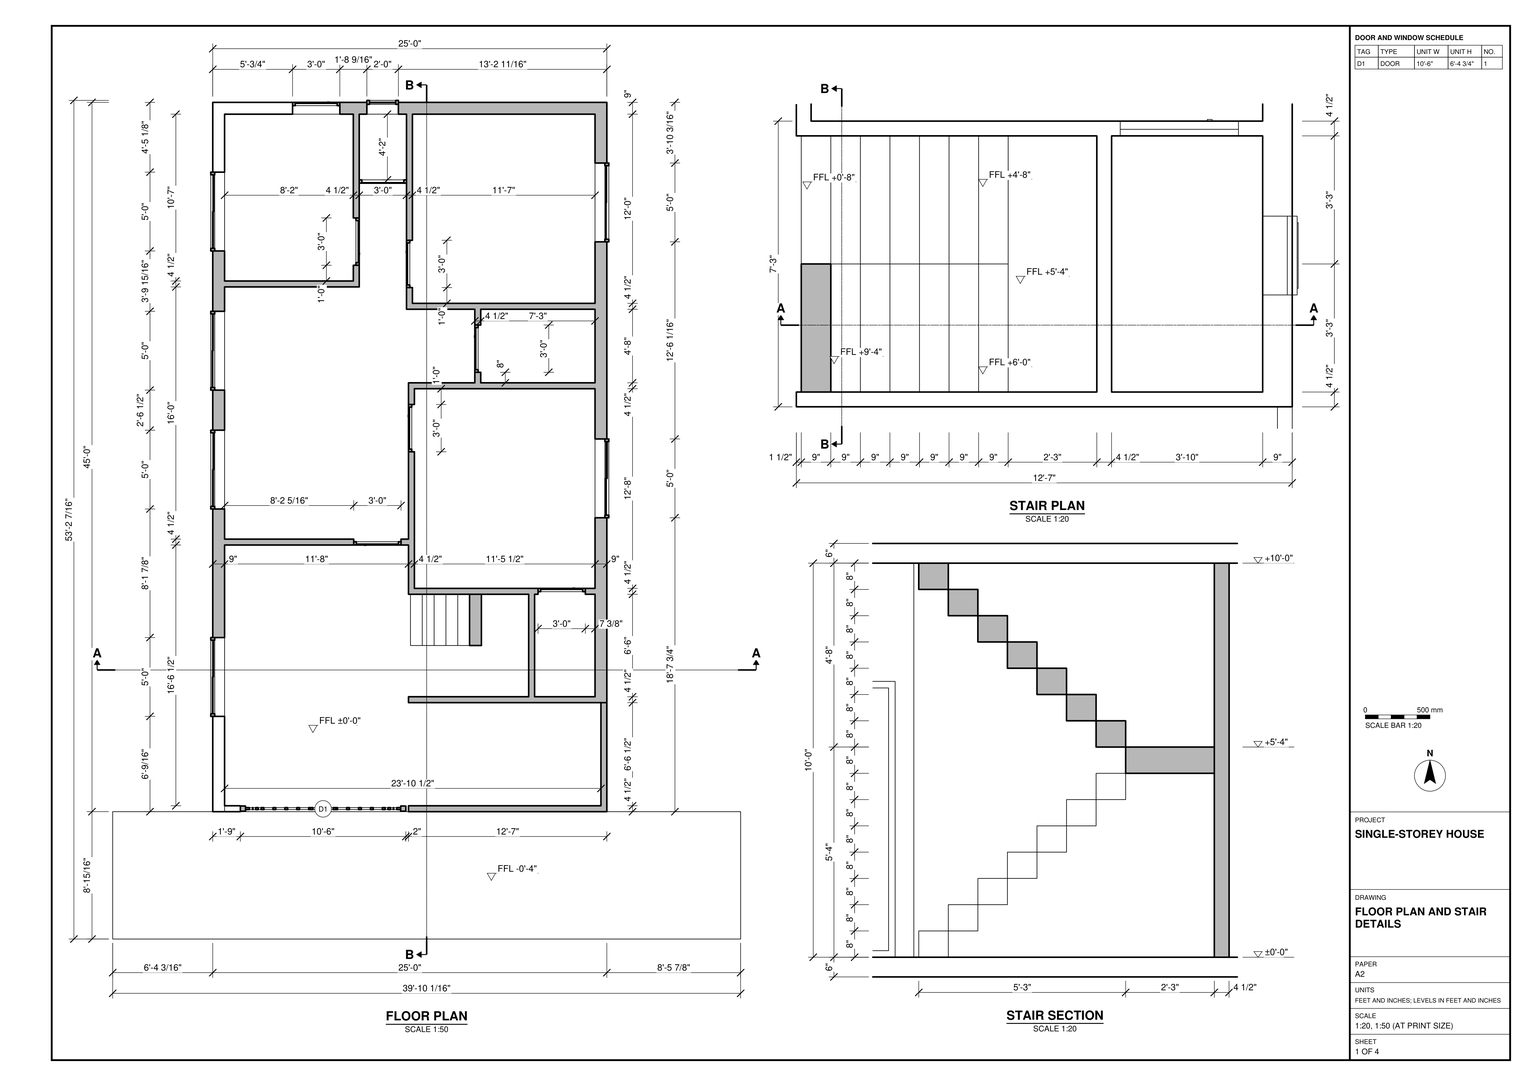
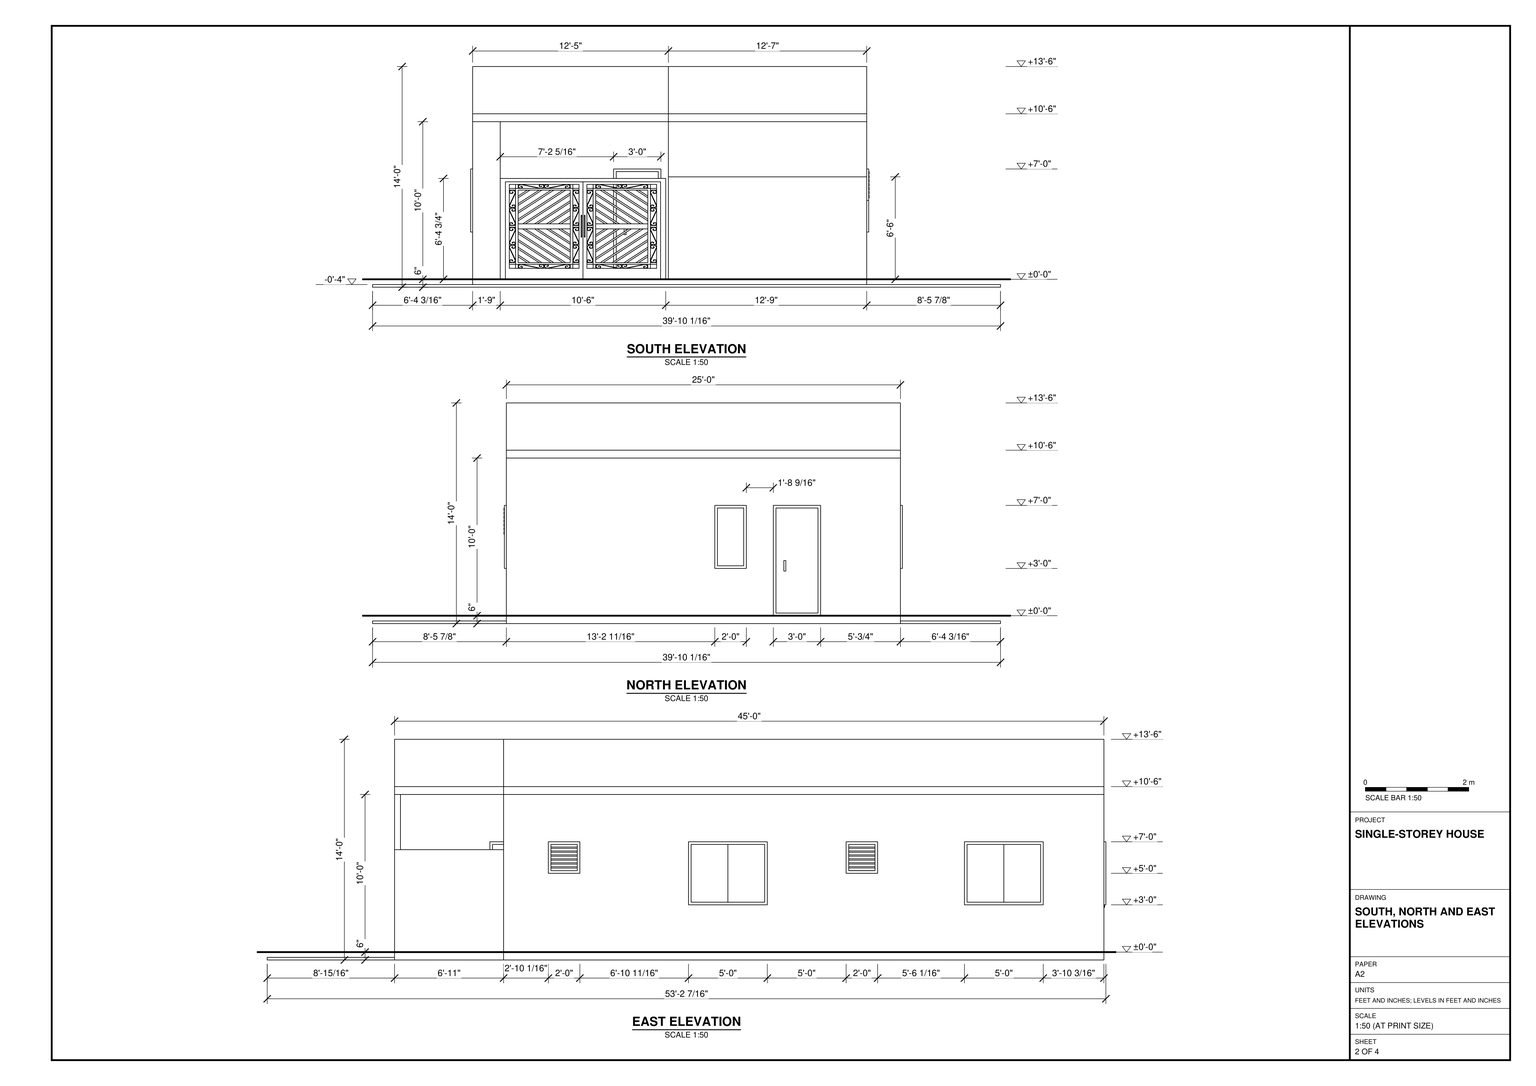
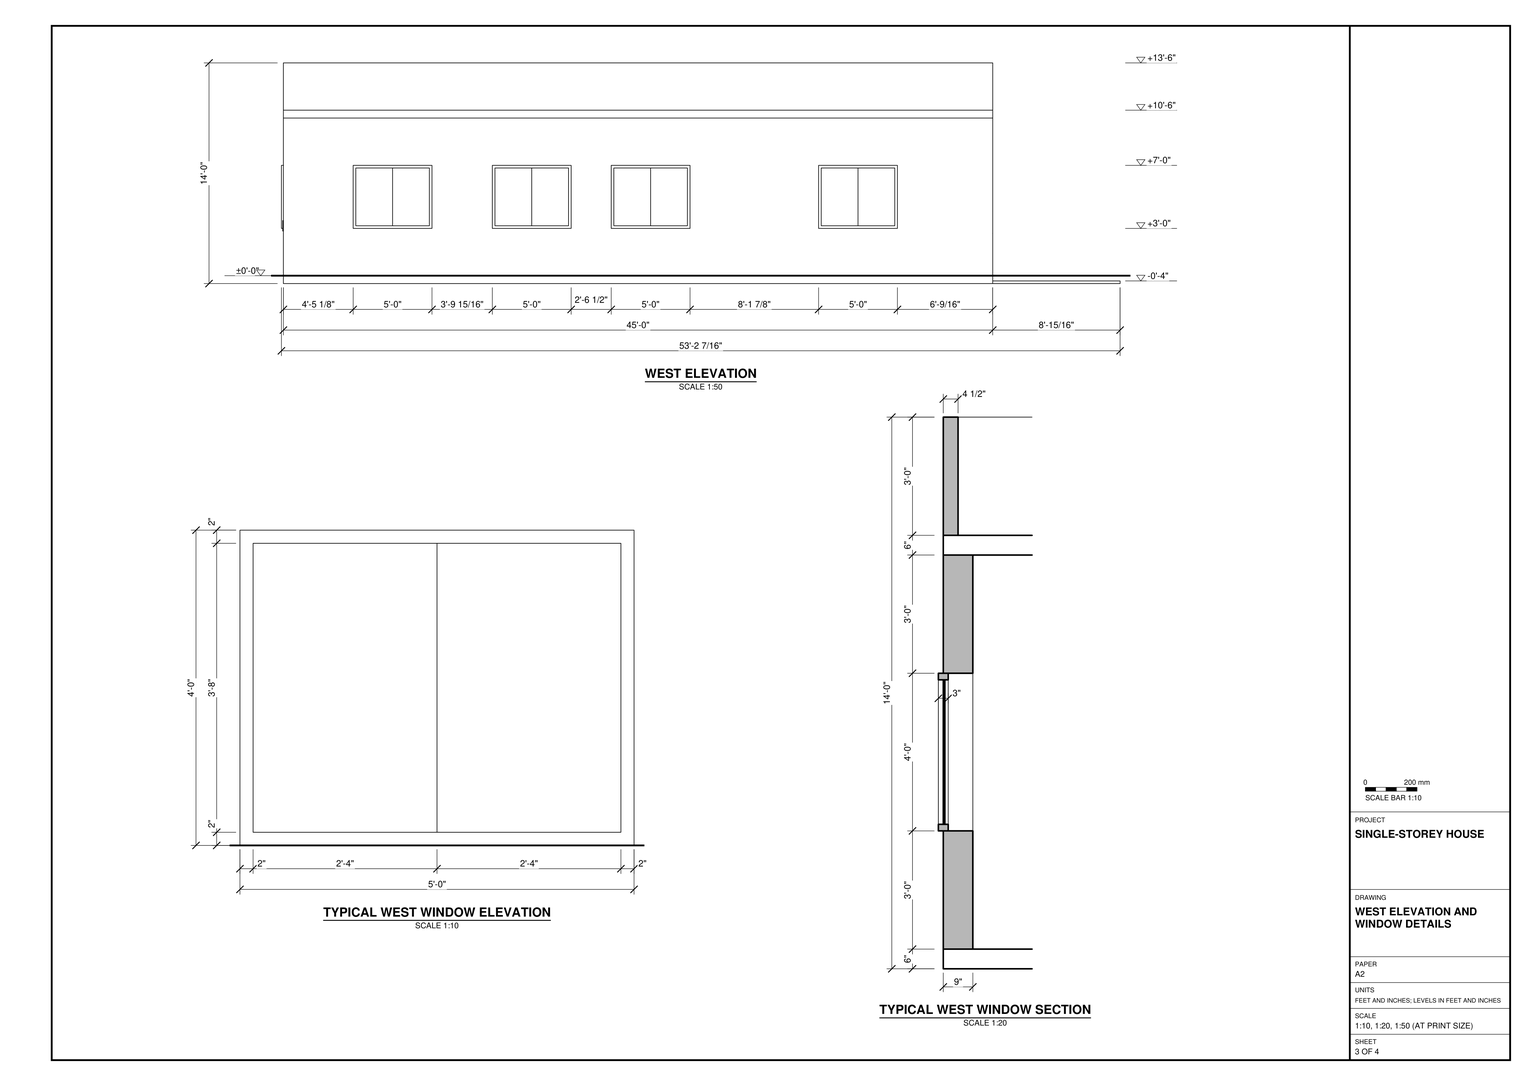
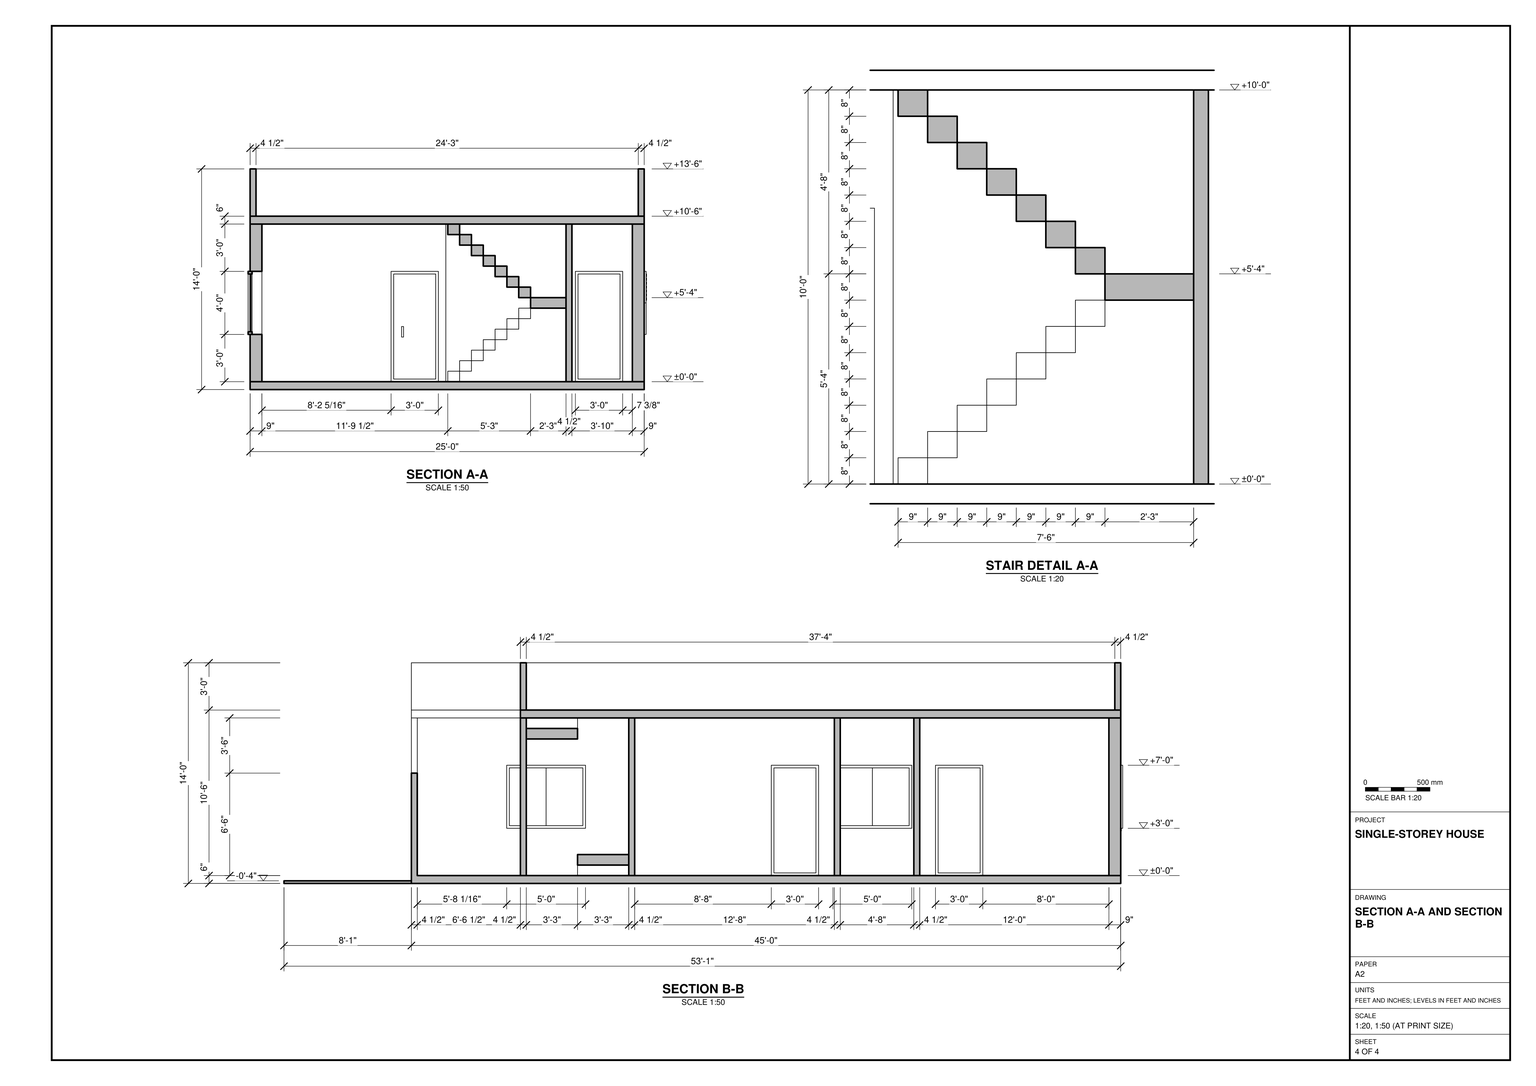
Build the single-storey house in SketchUp from task_files/diagram_01.pdf. Work in feet and inches. Set the ground floor at ±0'-0". The complete model, including the apron outside the south entrance, measures 39'-10 1/16" east to west, 53'-2 7/16" north to south and 14'-0" high. The house itself has a 25'-0" by 45'-0" footprint. Set the apron surface at -0'-4" and extend it past both sides of the house as shown in plan.

Model the floor slab, exterior walls and interior partitions, following the thicknesses and doorway positions on the plan. Preserve the open entrance area, the stair near its east side and the passage connecting the rooms farther north. Build the two stair flights and their intermediate landing from the stair plan and section. Model the flat roof slab and raised perimeter parapet. Fit the south entrance with the paired gate leaves shown in elevation. Use the window detail for the divided west windows, and distinguish the smaller louvred openings from the larger glazed windows on the east wall.

Keep shell elements such as walls, slabs and roof, and each furniture or joinery piece shown, in separate groups or components; use components for repeated parts. Any decor or loose items shown may be suitable library components. Save one SketchUp model as output_files/gated_single_storey_house_with_return_stair.skp.

# SketchUp Ruby script. Lengths in inches.
U = 1.inch
M = Sketchup.active_model
def pt(a) = Geom::Point3d.new(a.map { |v| v * U })
def face(e, loops, mat)
  f = e.add_face(loops[0].map { |a| pt(a) })
  loops[1..].each { |l| e.add_face(l.map { |a| pt(a) }).erase! }
  f.material = f.back_material = mat if mat
  f
end
# faces: each face lists its corners as indices into pts; further lists are holes
def faces(e, pts, list, mat = nil) = list.each { |f| face(e, (f[0].is_a?(Array) ? f : [f]).map { |l| l.map { |i| pts[i] } }, mat) }
# xy, xz, yz: faces in a plane at the given z, y or x. An outline is a flat list of corners, or four numbers for a rectangle; further outlines are holes
def ring(l) = l.size == 4 ? [[l[0], l[1]], [l[2], l[1]], [l[2], l[3]], [l[0], l[3]]] : l.each_slice(2).to_a
def flat(e, list, mat, &to3) = list.each { |f| face(e, (f[0].is_a?(Array) ? f : [f]).map { |l| ring(l).map { |u, v| to3.(u, v) } }, mat) }
def xy(e, z, list, mat = nil) = flat(e, list, mat) { |x, y| [x, y, z] }
def xz(e, y, list, mat = nil) = flat(e, list, mat) { |x, z| [x, y, z] }
def yz(e, x, list, mat = nil) = flat(e, list, mat) { |y, z| [x, y, z] }
def lines(e, pts, list) = list.each { |a, b| e.add_line(pt(pts[a]), pt(pts[b])) }
# prism: a flat outline (further loops are holes) pulled along v
def prism(e, loops, v, mat = nil)
  f = face(e, loops, mat); d = Geom::Vector3d.new(v.map { |x| x * U })
  f.pushpull(f.normal.samedirection?(d) ? d.length : -d.length)
end
def box(e, o, s, mat = nil) = prism(e, [[o, [o[0] + s[0], o[1], o[2]], [o[0] + s[0], o[1] + s[1], o[2]], [o[0], o[1] + s[1], o[2]]]], [0, 0, s[2]], mat)
def at(x, y, z, deg = 0) = Geom::Transformation.translation(pt([x, y, z])) * Geom::Transformation.rotation(ORIGIN, Z_AXIS, deg.degrees)
def axes(o, x, y, z) = Geom::Transformation.new([*x, 0, *y, 0, *z, 0, *pt(o).to_a, 1])
def part(name) = M.definitions.add(name)
# library, detail: a bought-in or finely detailed component or shape, given as its bounding box
def library(name, o, s) = part(name).tap { |d| box(d.entities, o, s) }
def detail(e, o, s) = box(e.add_group.entities, o, s)
def put(e, d, t, mat = nil) = e.add_instance(d, t).tap { |i| i.material = mat if mat }
def group(e, t, mat = nil) = e.add_group.tap { |g| g.transformation = t; g.material = mat if mat }.entities
root = M.entities
M.materials.add("Asphalt A02 100cm").color = [81, 81, 83]
M.materials.add("Glass Thin Clear 001").color = [0, 0, 0]
M.materials["Glass Thin Clear 001"].alpha = 0.1
M.materials.add("Metal Sandblasted Black 200cm").color = [86, 90, 95]
M.materials.add("Porcelain Dusk Blue Glossy Rough 001").color = [122, 143, 157]
M.materials.add("Porcelain SSS 001").color = [245, 243, 236]
M.materials["Porcelain SSS 001"].alpha = 0.6875
M.materials.add("Two Color Maple Panels 300cm").color = [56, 46, 41]
c1 = library("gate 271k",[0,0,0],[125.98,4.3125,118.11])
c2 = part("Group\#3")
box(c2.entities,[0,0,0],[0.31,28,44])
c3 = part("Group\#5")
box(c3.entities,[0,0,0],[0.31,28,44])
c4 = part("Group\#7")
box(c4.entities,[0,0,0],[0.31,28,44])
c5 = part("Group\#9")
box(c5.entities,[0,0,0],[0.31,28,44])
c6 = part("Group\#11")
box(c6.entities,[0,0,0],[0.31,20,2])
c7 = part("Group\#13")
box(c7.entities,[-0.75,0,0],[0.75,28,44])
c8 = part("Group\#15")
box(c8.entities,[0,0,0],[0.31,20,2])
c9 = part("Group\#17")
box(c9.entities,[-0.31,0,0],[0.31,28,44])
c10 = part("Group\#44")
box(c10.entities,[0,0,0],[9,39,8])
put(root,c1,axes([97.1875,96.96,0],[1,0,0],[0,1,0],[0,0,0.65]))
g1 = group(root,at(76.1875,96.96,0))
xy(g1,0,[[9,0,21,4.5],[60.75,531,96.75,540]])
xy(g1,36,[[0,72.5625,9,132.5625],[291,223.75,300,283.75],[0,230.4375,9,290.4375],[0,320.9375,9,380.9375],[0,426.875,9,486.875],
  [291,433.8125,300,493.8125],[117.3125,531,141.3125,540]])
xy(g1,60,[[291,117.0625,300,141.0625],[291,343.75,300,367.75]])
xy(g1,84,[[0,72.5625,9,132.5625],[291,117.0625,300,141.0625],[247.625,165.5,283.625,170],[107.3125,203,143.3125,207.5],[291,223.75,300,283.75],
  [0,230.4375,9,290.4375],[149,274,153.5,310],[0,320.9375,9,380.9375],[199.5,334.5,204,370.5],[291,343.75,300,367.75],
  [147.5,399,152,435],[107,416,111.5,452],[0,426.875,9,486.875],[291,433.8125,300,493.8125],[111.5,478.5,147.5,483],
  [60.75,531,96.75,540],[117.3125,531,141.3125,540]])
xy(g1,120,[[[0,0,21,0,21,4.5,9,4.5,9,203,149,203,149,165.5,240.5,165.5,240.5,87.5,149,87.5,149,83,300,83,300,540,0,540],[9,207.5,9,399.5,111.5,399.5,111.5,478.5,147.5,478.5,147.5,382.5,199.5,382.5,199.5,326.5,149,326.5,149,207.5],[153.5,170,291,322],[152,387,291,531],[9,404,107,531],[204,326.5,291,382.5],[245,87.5,291,165.5],[111.5,483,147.5,531]]])
xz(g1,0,[[0,0,21,120]],"Porcelain Dusk Blue Glossy Rough 001")
xz(g1,4.5,[[9,0,21,120]])
xz(g1,72.5625,[[0,36,9,84]])
xz(g1,83,[[149,0,300,120]],"Porcelain Dusk Blue Glossy Rough 001")
xz(g1,87.5,[[149,0,240.5,120],[245,0,291,120]])
xz(g1,117.0625,[[291,60,300,84]])
xz(g1,132.5625,[[0,36,9,84]])
xz(g1,141.0625,[[291,60,300,84]])
xz(g1,165.5,[[245,0,247.625,0,247.625,84,283.625,84,283.625,0,291,0,291,120,245,120]])
xz(g1,165.5,[[149,0,240.5,120]],"Porcelain Dusk Blue Glossy Rough 001")
xz(g1,170,[[153.5,0,153.5,120,291,120,291,0,283.625,0,283.625,84,247.625,84,247.625,0]])
xz(g1,203,[[9,0,107.3125,0,107.3125,84,143.3125,84,143.3125,0,149,0,149,120,9,120]],"Porcelain Dusk Blue Glossy Rough 001")
xz(g1,207.5,[[9,0,9,120,149,120,149,0,143.3125,0,143.3125,84,107.3125,84,107.3125,0]])
xz(g1,223.75,[[291,36,300,84]])
xz(g1,230.4375,[[0,36,9,84]])
xz(g1,274,[[149,0,153.5,84]])
xz(g1,283.75,[[291,36,300,84]])
xz(g1,290.4375,[[0,36,9,84]])
xz(g1,310,[[149,0,153.5,84]])
xz(g1,320.9375,[[0,36,9,84]])
xz(g1,322,[[153.5,0,291,120]])
xz(g1,326.5,[[149,0,199.5,120],[204,0,291,120]])
xz(g1,334.5,[[199.5,0,204,84]])
xz(g1,343.75,[[291,60,300,84]])
xz(g1,367.75,[[291,60,300,84]])
xz(g1,370.5,[[199.5,0,204,84]])
xz(g1,380.9375,[[0,36,9,84]])
xz(g1,382.5,[[147.5,0,199.5,120],[204,0,291,120]])
xz(g1,387,[[152,0,291,120]])
xz(g1,399,[[147.5,0,152,84]])
xz(g1,399.5,[[9,0,111.5,120]])
xz(g1,404,[[9,0,107,120]])
xz(g1,416,[[107,0,111.5,84]])
xz(g1,426.875,[[0,36,9,84]])
xz(g1,433.8125,[[291,36,300,84]])
xz(g1,435,[[147.5,0,152,84]])
xz(g1,452,[[107,0,111.5,84]])
xz(g1,478.5,[[111.5,84,147.5,120]])
xz(g1,483,[[111.5,84,147.5,120]])
xz(g1,486.875,[[0,36,9,84]])
xz(g1,493.8125,[[291,36,300,84]])
xz(g1,531,[[9,0,60.75,0,60.75,84,96.75,84,96.75,0,107,0,107,120,9,120],[[111.5,0,147.5,120],[117.3125,36,141.3125,84]],[152,0,291,120]])
xz(g1,540,[[[0,0,0,120,300,120,300,0,96.75,0,96.75,84,60.75,84,60.75,0],[117.3125,36,141.3125,84]]],"Porcelain Dusk Blue Glossy Rough 001")
yz(g1,0,[[[0,0,540,120],[72.5625,36,132.5625,84],[230.4375,36,290.4375,84],[320.9375,36,380.9375,84],[426.875,36,486.875,84]]],"Porcelain Dusk Blue Glossy Rough 001")
yz(g1,9,[[[207.5,0,399.5,120],[230.4375,36,290.4375,84],[320.9375,36,380.9375,84]],[[404,0,531,120],[426.875,36,486.875,84]]])
yz(g1,9,[[[4.5,0,203,120],[72.5625,36,132.5625,84]]],"Porcelain Dusk Blue Glossy Rough 001")
yz(g1,21,[[0,0,4.5,120]])
yz(g1,60.75,[[531,0,540,84]])
yz(g1,96.75,[[531,0,540,84]])
yz(g1,107,[[404,0,404,120,531,120,531,0,452,0,452,84,416,84,416,0]])
yz(g1,107.3125,[[203,0,207.5,84]])
yz(g1,111.5,[[399.5,0,416,0,416,84,452,84,452,0,531,0,531,120,483,120,483,84,478.5,84,478.5,120,399.5,120]])
yz(g1,117.3125,[[531,36,540,84]])
yz(g1,141.3125,[[531,36,540,84]])
yz(g1,143.3125,[[203,0,207.5,84]])
yz(g1,147.5,[[382.5,0,382.5,120,478.5,120,478.5,84,483,84,483,120,531,120,531,0,435,0,435,84,399,84,399,0]])
yz(g1,149,[[83,0,87.5,120],[207.5,0,207.5,120,326.5,120,326.5,0,310,0,310,84,274,84,274,0]])
yz(g1,149,[[165.5,0,203,120]],"Porcelain Dusk Blue Glossy Rough 001")
yz(g1,152,[[387,0,399,0,399,84,435,84,435,0,531,0,531,120,387,120]])
yz(g1,153.5,[[170,0,274,0,274,84,310,84,310,0,322,0,322,120,170,120]])
yz(g1,199.5,[[326.5,0,326.5,120,382.5,120,382.5,0,370.5,0,370.5,84,334.5,84,334.5,0]])
yz(g1,204,[[326.5,0,334.5,0,334.5,84,370.5,84,370.5,0,382.5,0,382.5,120,326.5,120]])
yz(g1,240.5,[[87.5,0,165.5,120]])
yz(g1,245,[[87.5,0,165.5,120]])
yz(g1,247.625,[[165.5,0,170,84]])
yz(g1,283.625,[[165.5,0,170,84]])
yz(g1,291,[[[87.5,0,165.5,120],[117.0625,60,141.0625,84]],[[170,0,322,120],[223.75,36,283.75,84]],[[326.5,0,382.5,120],[343.75,60,367.75,84]],[[387,0,531,120],[433.8125,36,493.8125,84]]])
yz(g1,300,[[[83,0,540,120],[433.8125,36,493.8125,84],[223.75,36,283.75,84],[343.75,60,367.75,84],[117.0625,60,141.0625,84]]],"Porcelain Dusk Blue Glossy Rough 001")
g2 = group(g1,at(0,426.875,36))
prism(g2,[[[-1.5,60,0],[-1.5,0,0],[-1.5,0,48],[-1.5,60,48]],[[-1.5,58,2],[-1.5,58,46],[-1.5,2,46],[-1.5,2,2]]],[3,0,0],"Metal Sandblasted Black 200cm")
put(g2,c2,at(0.3125,30,2),"Glass Thin Clear 001")
put(g2,c2,at(0,2,2),"Glass Thin Clear 001")
g3 = group(g1,at(0,320.9375,36))
prism(g3,[[[-1.5,60,0],[-1.5,0,0],[-1.5,0,48],[-1.5,60,48]],[[-1.5,2,2],[-1.5,58,2],[-1.5,58,46],[-1.5,2,46]]],[3,0,0],"Metal Sandblasted Black 200cm")
put(g3,c3,at(-0.0625,30,2),"Glass Thin Clear 001")
put(g3,c3,at(-0.38,2,2),"Glass Thin Clear 001")
g4 = group(g1,at(0,230.4375,36))
prism(g4,[[[-1.5,60,0],[-1.5,0,0],[-1.5,0,48],[-1.5,60,48]],[[-1.5,2,2],[-1.5,58,2],[-1.5,58,46],[-1.5,2,46]]],[3,0,0],"Metal Sandblasted Black 200cm")
put(g4,c4,at(0.3125,30,2),"Glass Thin Clear 001")
put(g4,c4,at(0,2,2),"Glass Thin Clear 001")
g5 = group(g1,at(0,72.5625,36))
prism(g5,[[[-1.5,60,0],[-1.5,0,0],[-1.5,0,48],[-1.5,60,48]],[[-1.5,58,46],[-1.5,2,46],[-1.5,2,2],[-1.5,58,2]]],[3,0,0],"Metal Sandblasted Black 200cm")
put(g5,c5,at(0.125,30,2),"Glass Thin Clear 001")
put(g5,c5,at(-0.19,2,2),"Glass Thin Clear 001")
g6 = group(g1,at(300,117.0625,60))
prism(g6,[[[1.5,0,0],[1.5,24,0],[1.5,24,24],[1.5,0,24]],[[1.5,2,2],[1.5,2,22],[1.5,22,22],[1.5,22,2]]],[-3,0,0],"Metal Sandblasted Black 200cm")
put(g6,c6,at(1.5,2,20),"Glass Thin Clear 001")
put(g6,c6,at(1.5,2,17),"Glass Thin Clear 001")
put(g6,c6,at(1.5,2,14),"Glass Thin Clear 001")
put(g6,c6,at(1.5,2,11),"Glass Thin Clear 001")
put(g6,c6,at(1.5,2,8),"Glass Thin Clear 001")
put(g6,c6,at(1.5,2,5),"Glass Thin Clear 001")
put(g6,c6,at(1.5,2,2),"Glass Thin Clear 001")
g7 = group(g1,at(300,223.75,36))
prism(g7,[[[1.5,0,0],[1.5,60,0],[1.5,60,48],[1.5,0,48]],[[1.5,58,2],[1.5,2,2],[1.5,2,46],[1.5,58,46]]],[-3,0,0],"Metal Sandblasted Black 200cm")
put(g7,c7,at(-0.5,2,2),"Glass Thin Clear 001")
put(g7,c7,at(0.25,30,2),"Glass Thin Clear 001")
g8 = group(g1,at(300,343.75,60))
prism(g8,[[[1.5,0,0],[1.5,24,0],[1.5,24,24],[1.5,0,24]],[[1.5,2,2],[1.5,2,22],[1.5,22,22],[1.5,22,2]]],[-3,0,0],"Metal Sandblasted Black 200cm")
put(g8,c8,at(1.5,2,20),"Glass Thin Clear 001")
put(g8,c8,at(1.5,2,17.01),"Glass Thin Clear 001")
put(g8,c8,at(1.5,2,14.02),"Glass Thin Clear 001")
put(g8,c8,at(1.5,2,11.03),"Glass Thin Clear 001")
put(g8,c8,at(1.5,2,8.04),"Glass Thin Clear 001")
put(g8,c8,at(1.5,2,5.05),"Glass Thin Clear 001")
put(g8,c8,at(1.5,2,2.0625),"Glass Thin Clear 001")
g9 = group(g1,at(300,433.8125,36))
prism(g9,[[[1.5,0,0],[1.5,60,0],[1.5,60,48],[1.5,0,48]],[[1.5,2,2],[1.5,2,46],[1.5,58,46],[1.5,58,2]]],[-3,0,0],"Metal Sandblasted Black 200cm")
put(g9,c9,at(-0.625,2,2),"Glass Thin Clear 001")
put(g9,c9,at(-0.31,30,2),"Glass Thin Clear 001")
g10 = group(g1,at(117.3125,540,36))
prism(g10,[[[0,1.5,0],[0,1.5,48],[24,1.5,48],[24,1.5,0]],[[22,1.5,2],[22,1.5,46],[2,1.5,46],[2,1.5,2]]],[0,-3,0],"Metal Sandblasted Black 200cm")
g11 = group(g10,at(2,0,2),"Glass Thin Clear 001")
box(g11,[0,-0.31,0],[20,0.31,44])
g12 = group(g1,at(60.75,540,0))
prism(g12,[[[0,0,0],[0,0,84],[36,0,84],[36,0,0]],[[2,0,82],[2,0,2],[34,0,2],[34,0,82]]],[0,-2.5,0],"Metal Sandblasted Black 200cm")
g13 = group(g12,at(2,0,2))
box(g13,[0,-0.71,0],[32,0.71,80],"Two Color Maple Panels 300cm")
g14 = group(g13,at(26,0,32),"Metal Sandblasted Black 200cm")
box(g14,[-1.5,0,0],[1.5,0.5,8])
g15 = group(g1,at(107.3125,203,0))
prism(g15,[[[36,0,0],[36,0,84],[0,0,84],[0,0,0]],[[34,0,82],[34,0,2],[2,0,2],[2,0,82]]],[0,2.5,0],"Metal Sandblasted Black 200cm")
g16 = group(g15,at(2,0,2),"Two Color Maple Panels 300cm")
xy(g16,0,[[0,0,32,0.71]])
xy(g16,80,[[0,0,32,0.71]])
xz(g16,0,[[0,0,32,80]],"Two Color Maple Panels 300cm")
xz(g16,0.71,[[0,0,32,80]])
yz(g16,0,[[0,0,0.71,80]])
yz(g16,32,[[0,0,0.71,80]])
g17 = group(g16,at(6,0,32),"Metal Sandblasted Black 200cm")
box(g17,[0,-0.5,0],[1.5,0.5,8])
g18 = group(g1,at(149,274,0))
prism(g18,[[[0,0,0],[0,0,84],[0,36,84],[0,36,0]],[[0,2,2],[0,34,2],[0,34,82],[0,2,82]]],[2.5,0,0],"Metal Sandblasted Black 200cm")
g19 = group(g18,at(0,2,2))
box(g19,[0,0,0],[0.71,32,80],"Two Color Maple Panels 300cm")
g20 = group(g19,at(0,26,32),"Metal Sandblasted Black 200cm")
box(g20,[-0.5,-1.5,0],[0.5,1.5,8])
g21 = group(g1,at(199.5,334.5,0))
prism(g21,[[[0,0,0],[0,0,84],[0,36,84],[0,36,0]],[[0,2,2],[0,34,2],[0,34,82],[0,2,82]]],[2.5,0,0],"Metal Sandblasted Black 200cm")
g22 = group(g21,at(0,2,2))
box(g22,[0,0,0],[0.71,32,80],"Two Color Maple Panels 300cm")
g23 = group(g22,at(0,26,32),"Metal Sandblasted Black 200cm")
box(g23,[-0.5,-1.5,0],[0.5,1.5,8])
g24 = group(g1,at(147.5,399,0))
prism(g24,[[[0,0,0],[0,0,84],[0,36,84],[0,36,0]],[[0,34,2],[0,34,82],[0,2,82],[0,2,2]]],[2.5,0,0],"Metal Sandblasted Black 200cm")
g25 = group(g24,at(0,2,2))
box(g25,[0,0,0],[0.71,32,80],"Two Color Maple Panels 300cm")
g26 = group(g25,at(0,26,32),"Porcelain Dusk Blue Glossy Rough 001")
box(g26,[-0.5,-1.5,0],[0.5,1.5,8])
g27 = group(g1,at(111.5,416,0))
prism(g27,[[[0,36,0],[0,36,84],[0,0,84],[0,0,0]],[[0,34,82],[0,34,2],[0,2,2],[0,2,82]]],[-2.5,0,0],"Metal Sandblasted Black 200cm")
g28 = group(g27,at(0,2,2))
xy(g28,0,[[-0.71,0,0,32]])
xy(g28,80,[[-0.71,0,0,32]])
xz(g28,0,[[-0.71,0,0,80]])
xz(g28,32,[[-0.71,0,0,80]])
yz(g28,-0.71,[[0,0,32,80]],"Two Color Maple Panels 300cm")
yz(g28,0,[[0,0,32,80]],"Two Color Maple Panels 300cm")
g29 = group(g28,at(0,6,32),"Metal Sandblasted Black 200cm")
box(g29,[0,0,0],[0.5,1.5,8])
g30 = group(g1,at(111.5,478.5,0))
prism(g30,[[[36,0,0],[36,0,84],[0,0,84],[0,0,0]],[[34,0,82],[34,0,2],[2,0,2],[2,0,82]]],[0,2.5,0],"Metal Sandblasted Black 200cm")
g31 = group(g30,at(2,0,2))
box(g31,[0,0,0],[32,0.31,80],"Glass Thin Clear 001")
g32 = group(g1,at(247.625,170,0))
prism(g32,[[[0,0,0],[0,0,84],[36,0,84],[36,0,0]],[[2,0,82],[2,0,2],[34,0,2],[34,0,82]]],[0,-2.5,0],"Metal Sandblasted Black 200cm")
g33 = group(g32,at(2,0,2))
box(g33,[0,-0.71,0],[32,0.71,80],"Two Color Maple Panels 300cm")
g34 = group(g33,at(26,0,32),"Metal Sandblasted Black 200cm")
box(g34,[-1.5,0,0],[1.5,0.5,8])
put(root,c10,at(226.6875,223.46,0))
put(root,c10,at(235.6875,223.46,8))
put(root,c10,at(244.6875,223.46,16))
put(root,c10,at(253.6875,223.46,24))
put(root,c10,at(262.6875,223.46,32))
put(root,c10,at(271.6875,223.46,40))
put(root,c10,at(280.6875,223.46,48))
g35 = group(root,at(289.6875,223.46,56))
box(g35,[0,-39,0],[27,78,8])
put(root,c10,at(280.6875,184.46,64))
put(root,c10,at(271.6875,184.46,72))
put(root,c10,at(262.6875,184.46,80))
put(root,c10,at(253.6875,184.46,88))
put(root,c10,at(244.6875,184.46,96))
put(root,c10,at(235.6875,184.46,104))
put(root,c10,at(226.6875,184.46,112))
g36 = group(root,at(76.1875,179.96,120))
xy(g36,-126,[[0,-83,300,457]])
xy(g36,-120,[[0,-83,149,-83,149,-78.5,295.5,-78.5,295.5,0,300,0,300,457,0,457]])
xy(g36,-42,[[149,-83,300,-83,300,0,295.5,0,295.5,-78.5,149,-78.5]])
xy(g36,0,[[0,-83,0,457,300,457,300,0,149,0,149,-83]],"Porcelain Dusk Blue Glossy Rough 001")
xy(g36,6,[[4.5,-78.5,144.5,-78.5,144.5,4.5,295.5,4.5,295.5,452.5,4.5,452.5]])
xz(g36,-83,[[0,0,149,6]],"Porcelain Dusk Blue Glossy Rough 001")
xz(g36,-83,[[0,-126,300,-126,300,-42,149,-42,149,-120,0,-120]],"Porcelain SSS 001")
xz(g36,-78.5,[[149,-120,295.5,-42]])
xz(g36,0,[[295.5,-120,300,-42]])
xz(g36,0,[[149,0,300,6]],"Porcelain Dusk Blue Glossy Rough 001")
xz(g36,457,[[0,-126,300,-120]])
xz(g36,457,[[0,0,300,6]],"Porcelain Dusk Blue Glossy Rough 001")
yz(g36,0,[[-83,-126,457,-120]])
yz(g36,0,[[-83,0,457,6]],"Porcelain Dusk Blue Glossy Rough 001")
yz(g36,149,[[-83,-120,-78.5,-42]])
yz(g36,149,[[-83,0,0,6]],"Porcelain Dusk Blue Glossy Rough 001")
yz(g36,295.5,[[-78.5,-120,0,-42]])
yz(g36,300,[[0,-126,457,-120]])
yz(g36,300,[[0,0,457,6]],"Porcelain Dusk Blue Glossy Rough 001")
yz(g36,300,[[-83,-126,0,-42]],"Porcelain SSS 001")
p = [[149,0,-120],[295.5,0,-120]]
lines(g36,p,[[0,1]])
g37 = group(g36,at(0,-83,6),"Porcelain SSS 001")
prism(g37,[[[0,0,0],[0,540,0],[300,540,0],[300,83,0],[149,83,0],[149,0,0]],[[4.5,4.5,0],[144.5,4.5,0],[144.5,87.5,0],[295.5,87.5,0],[295.5,535.5,0],[4.5,535.5,0]]],[0,0,36],"Porcelain SSS 001")
g38 = group(root,at(76.1875,50.6875,-6),"Asphalt A02 100cm")
box(g38,[-76.1875,-50.6875,0],[478.04,96.96,2],"Asphalt A02 100cm")
